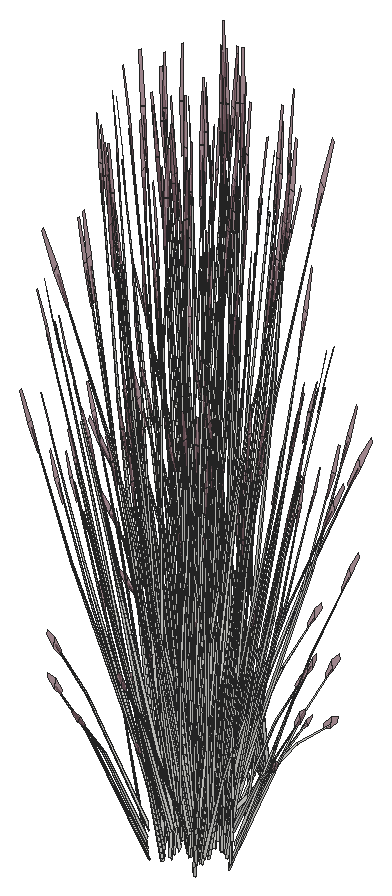
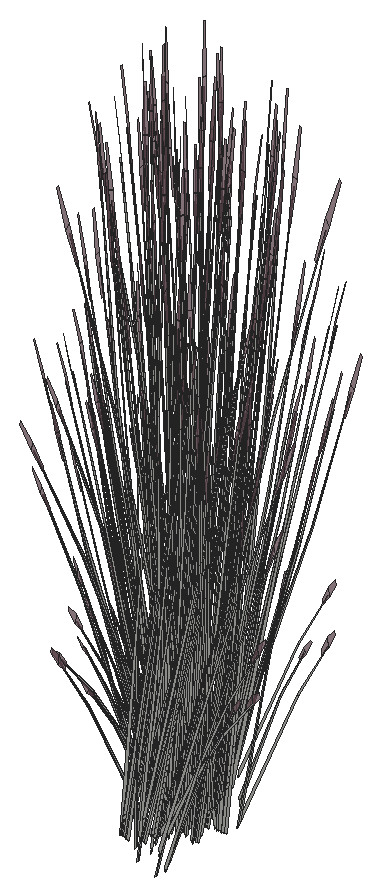
# SketchUp Ruby script. Lengths in inches.
U = 1.inch
M = Sketchup.active_model
def pt(a) = Geom::Point3d.new(a.map { |v| v * U })
def face(e, loops, mat)
  f = e.add_face(loops[0].map { |a| pt(a) })
  loops[1..].each { |l| e.add_face(l.map { |a| pt(a) }).erase! }
  f.material = f.back_material = mat if mat
  f
end
# faces: each face lists its corners as indices into pts; further lists are holes
def faces(e, pts, list, mat = nil) = list.each { |f| face(e, (f[0].is_a?(Array) ? f : [f]).map { |l| l.map { |i| pts[i] } }, mat) }
# xy, xz, yz: faces in a plane at the given z, y or x. An outline is a flat list of corners, or four numbers for a rectangle; further outlines are holes
def ring(l) = l.size == 4 ? [[l[0], l[1]], [l[2], l[1]], [l[2], l[3]], [l[0], l[3]]] : l.each_slice(2).to_a
def flat(e, list, mat, &to3) = list.each { |f| face(e, (f[0].is_a?(Array) ? f : [f]).map { |l| ring(l).map { |u, v| to3.(u, v) } }, mat) }
def xy(e, z, list, mat = nil) = flat(e, list, mat) { |x, y| [x, y, z] }
def xz(e, y, list, mat = nil) = flat(e, list, mat) { |x, z| [x, y, z] }
def yz(e, x, list, mat = nil) = flat(e, list, mat) { |y, z| [x, y, z] }
def lines(e, pts, list) = list.each { |a, b| e.add_line(pt(pts[a]), pt(pts[b])) }
# prism: a flat outline (further loops are holes) pulled along v
def prism(e, loops, v, mat = nil)
  f = face(e, loops, mat); d = Geom::Vector3d.new(v.map { |x| x * U })
  f.pushpull(f.normal.samedirection?(d) ? d.length : -d.length)
end
def box(e, o, s, mat = nil) = prism(e, [[o, [o[0] + s[0], o[1], o[2]], [o[0] + s[0], o[1] + s[1], o[2]], [o[0], o[1] + s[1], o[2]]]], [0, 0, s[2]], mat)
def at(x, y, z, deg = 0) = Geom::Transformation.translation(pt([x, y, z])) * Geom::Transformation.rotation(ORIGIN, Z_AXIS, deg.degrees)
def axes(o, x, y, z) = Geom::Transformation.new([*x, 0, *y, 0, *z, 0, *pt(o).to_a, 1])
def part(name) = M.definitions.add(name)
# library, detail: a bought-in or finely detailed component or shape, given as its bounding box
def library(name, o, s) = part(name).tap { |d| box(d.entities, o, s) }
def detail(e, o, s) = box(e.add_group.entities, o, s)
def put(e, d, t, mat = nil) = e.add_instance(d, t).tap { |i| i.material = mat if mat }
def group(e, t, mat = nil) = e.add_group.tap { |g| g.transformation = t; g.material = mat if mat }.entities
root = M.entities
M.materials.add("LightPink_Translucent").color = [144, 107, 117]
M.materials["LightPink_Translucent"].alpha = 0.75
c1 = part("blade")
p = [[2.15,0.21,22],[0,0.17,0],[0.09,0.45,0],[2.18,0.31,22],[2.29,0.31,22],[0.38,0.45,0],
  [2.48,0.24,33],[2.49,0.24,33],[2.48,0.22,33]]
faces(c1.entities,p,[[0,1,2,3],[4,5,2,3],[6,3,4,7],[8,0,3,6]])
c2 = part("seeds")
p = [[0.3,-0.1,1.38],[-0.01,-0.03,1.59],[-0.01,-0.03,0.03],[0.14,-0.07,-0.07],[0.29,-0.03,3],[0.15,0.01,3.11]]
faces(c2.entities,p,[[0,1,2,3],[1,0,4,5]],"LightPink_Translucent")
c3 = part("blade with seeds")
put(c3.entities,c1,at(0,0,0))
put(c3.entities,c2,axes([2.4,0.25,30.99],[1.5799,-0.05474,1.17369],[-0.12525,1.92788,0.29478],[-0.07173,-0.02425,1.56792]))
put(root,c3,axes([413.03,278.98,-8.39],[-0.09522,0.18683,1.59586],[-0.39947,-0.38663,0.12904],[0.18021,-0.24097,0.68222]))
put(root,c3,axes([414.33,278.06,-7.62],[-0.05194,0.04152,1.65179],[-0.50886,-0.14007,-0.15608],[-0.01842,-0.18118,0.29231]))
put(root,c3,axes([412.46,278.72,-7.64],[-0.50273,-0.13626,-0.47583],[0.17232,-0.46717,-0.36857],[-0.0461,-0.18809,0.91046]))
put(root,c3,axes([412.77,277.55,-9.42],[0.06561,0.31695,1.06958],[-0.36394,-0.17555,0.78586],[0.03916,-0.16229,0.23558]))
put(root,c3,axes([413.55,279.07,-7.64],[-0.3661,-0.36521,-0.47583],[0.38674,-0.31985,-0.36857],[0.0557,-0.18556,0.91046]))
put(root,c3,axes([411.5625,277.27,-7.62],[-0.00954,0.06515,1.65179],[-0.47055,0.23645,-0.15608],[-0.13847,-0.12087,0.29231]))
put(root,c3,axes([411.46,278.43,-7.26],[0.56969,-0.13971,0.50064],[0.09887,0.54803,0.4128],[-0.13398,-0.16152,1.03595]))
put(root,c3,axes([412.75,278.53,-7.59],[0.50393,0.1421,0.447],[-0.17232,0.46717,0.36857],[-0.03028,-0.18372,0.92496]))
put(root,c3,axes([412.89,278.7,-7.3125],[-0.50045,0.25306,-0.11324],[-0.24593,-0.44915,-0.62851],[-0.06603,-0.18927,0.95501]))
put(root,c3,axes([413.93,279.26,-7.3125],[-0.56206,-0.02693,-0.11324],[0.01536,-0.50991,-0.62851],[0.03904,-0.19638,0.95501]))
put(root,c3,axes([413.89,278.9375,-7.78],[0.34603,-0.28618,-0.32977],[0.32756,0.32677,0.42575],[0.04984,-0.16603,0.81462]))
put(root,c3,axes([410.9,277.93,-9.42],[0.26677,0.18918,1.06958],[-0.38851,0.11372,0.78586],[-0.08313,-0.14539,0.23558]))
put(root,c3,axes([412.88,278.49,-7.6],[0.37684,-0.18473,0.05988],[0.18445,0.33686,0.47138],[-0.03639,-0.14849,0.71878]))
put(root,c3,axes([411.54,278.93,-7.36],[-0.43608,-0.26272,-0.66157],[0.30991,-0.46038,0.07984],[-0.158,-0.15687,0.93586]))
put(root,c3,axes([411.39,278.58,-7.78],[-0.07899,-0.43781,-0.32977],[0.45153,-0.11561,0.42575],[-0.12128,-0.12546,0.81462]))
put(root,c3,axes([411.59,278.54,-7.6],[0.23243,-0.34529,0.05988],[0.331,0.20103,0.47138],[-0.10701,-0.1107,0.71878]))
put(root,c3,axes([410.69,278.5,-10.61],[-0.04954,0.0716,1.6421],[-0.50062,0.15438,-0.25086],[-0.12094,-0.14044,0.2797]))
put(root,c3,axes([411.52,280.47,-10.05],[-0.21003,-0.55738,-0.65031],[0.60499,-0.20074,-0.17068],[-0.02321,-0.18874,1.43544]))
put(root,c3,axes([414.32,278.76,-10.61],[-0.07655,-0.04282,1.6421],[-0.19662,-0.47839,-0.25086],[0.13264,-0.12982,0.2797]))
put(root,c3,axes([412.74,278.87,-7.3],[-0.15418,0.41799,0.32977],[-0.44981,-0.12192,-0.42575],[-0.04124,-0.16829,0.81462]))
put(root,c3,axes([411.34,278.94,-7.64],[-0.50465,0.12921,-0.47583],[-0.08828,-0.48932,-0.36857],[-0.13555,-0.14022,0.91046]))
put(root,c3,axes([413.89,279.05,-7.59],[0.36417,0.37086,0.447],[-0.38674,0.31985,0.36857],[0.06718,-0.174,0.92496]))
put(root,c3,axes([411.69,278.51,-6.94],[-0.34131,0.52108,-0.12682],[-0.49429,-0.3002,-0.70393],[-0.17182,-0.14722,1.06961]))
put(root,c3,axes([414.02,279.08,-7.6],[0.42027,0.02533,0.05988],[-0.01152,0.38243,0.47138],[0.04398,-0.14649,0.71878]))
put(root,c3,axes([413.71,279.34,-7.3],[-0.34603,0.28618,0.32977],[-0.32756,-0.32677,-0.42575],[0.04984,-0.16603,0.81462]))
put(root,c3,axes([414.32,280.11,-7.36],[0.26714,-0.42887,-0.66157],[0.46811,0.30479,0.07984],[0.1595,-0.15539,0.93586]))
put(root,c3,axes([411.43,278.86,-9.79],[-0.31974,-0.54466,0],[0.53494,-0.30375,-0.48057],[0.12184,-0.06918,1.52448]))
put(root,c3,axes([414.31,279.91,-7.64],[-0.13138,-0.49631,-0.47583],[0.49754,-0.08682,-0.36857],[0.14258,-0.13331,0.91046]))
put(root,c3,axes([412.14,278.21,-10.02],[-0.35341,0.31182,-0.03625],[-0.32382,-0.34152,-0.16435],[-0.0228,-0.09677,0.54209]))
put(root,c3,axes([414.54,280.27,-7.3125],[-0.47307,-0.29971,-0.11324],[0.27254,-0.43404,-0.62851],[0.13365,-0.15087,0.95501]))
put(root,c3,axes([412.59,281.9,-8.9],[0.44194,0.21918,1.40854],[-0.43295,0.47219,0.557],[-0.19393,-0.27986,1.18082]))
put(root,c3,axes([411.66,278.94,-7.3],[0.07899,0.43781,0.32977],[-0.45153,0.11561,-0.42575],[-0.12128,-0.12546,0.81462]))
put(root,c3,axes([410.28,280.39,-10.12],[0,-0.54355,-0.46235],[0.57217,0,0],[0,-0.1238,1.46668]))
put(root,c3,axes([411.87,278.78,-10.12],[0.47863,-0.27177,-0.46235],[0.28609,0.48733,0],[0.10901,-0.0619,1.46668]))
put(root,c3,axes([414.71,279.72,-9.59],[-0.1827,-0.0161,1.33163],[-0.18717,-0.43188,-0.28638],[0.22444,-0.12218,0.56934]))
put(root,c3,axes([410.3,279.23,-7.26],[0.42234,-0.40113,0.50064],[0.36424,0.42599,0.4128],[-0.19815,-0.07399,1.03595]))
put(root,c3,axes([415.71,280.14,-7.62],[-0.0668,-0.00413,1.65179],[-0.27738,-0.44233,-0.15608],[0.11139,-0.14544,0.29231]))
put(root,c3,axes([412.44,279.89,-10.08],[0.34446,-0.40855,-0.58063],[0.42791,0.37046,-0.15239],[0.13803,-0.10191,1.28164]))
put(root,c3,axes([414.92,278.92,-9.42],[-0.17034,0.27669,1.06958],[-0.14642,-0.37174,0.78586],[0.14069,-0.09315,0.23558]))
put(root,c3,axes([414.68,279.96,-7.78],[0.44516,-0.07768,-0.32977],[0.11755,0.44407,0.42575],[0.12757,-0.11927,0.81462]))
put(root,c3,axes([410.5,279.22,-7.6],[0.02575,-0.41332,0.05988],[0.38885,0.01133,0.47138],[-0.14895,-0.04325,0.71878]))
put(root,c3,axes([411.84,280.61,-9.94],[0.24813,-0.48978,-0.41661],[0.51557,0.23571,0.2005],[0,-0.1129,1.33761]))
put(root,c3,axes([412.0625,280.37,-9.52],[-0.05959,-0.62022,-0.27094],[0.62068,-0.0375,-0.46562],[0.1093,-0.08261,1.4872]))
put(root,c3,axes([410.52,280.4,-10.11],[0.35699,-0.33913,-0.28847],[0.35699,0.33913,0.28847],[0,-0.10923,1.29413]))
put(root,c3,axes([410.38,278.77,-10.02],[-0.14753,0.44383,-0.03625],[-0.45406,-0.13653,-0.16435],[-0.06894,-0.07259,0.54209]))
put(root,c3,axes([414.3125,280.23,-7.3],[-0.44516,0.07768,0.32977],[-0.11755,-0.44407,-0.42575],[0.12757,-0.11927,0.81462]))
put(root,c3,axes([411.77,281.02,-9.52],[-0.57594,-0.25935,-0.27094],[0.27732,-0.5474,-0.46562],[-0.0181,-0.1344,1.4872]))
put(root,c3,axes([410.13,280.8,-9.79],[-0.63949,0,0],[0,-0.60749,-0.48057],[0,-0.13836,1.52448]))
put(root,c3,axes([411.98,278.99,-10.11],[0.47712,0.13449,-0.28847],[-0.12013,0.47362,0.28847],[0.09619,-0.05462,1.29413]))
put(root,c3,axes([414.72,280.16,-7.6],[0.35109,0.22859,0.05988],[-0.2044,0.32553,0.47138],[0.11256,-0.10524,0.71878]))
put(root,c3,axes([414.62,280.06,-7.59],[0.12683,0.50025,0.447],[-0.49754,0.08682,0.36857],[0.14663,-0.11765,0.92496]))
put(root,c3,axes([415.96,280.67,-7.61],[0.07097,-0.08279,1.62908],[-0.09083,-0.50786,-0.25764],[0.17806,-0.09629,0.13065]))
put(root,c3,axes([410.63,280.64,-9.83],[-0.47569,0.45698,0.2864],[-0.47598,-0.45217,-0.33981],[-0.01661,-0.12977,1.53541]))
put(root,c3,axes([412.14,280.85,-9.73],[0.57623,0.26344,0.22409],[-0.27732,0.5474,0.46562],[0,-0.12618,1.49497]))
put(root,c3,axes([411.92,281.59,-9.73],[0.13555,-0.64407,-0.21817],[0.64269,0.11227,0.47743],[-0.1123,-0.08895,1.45677]))
put(root,c3,axes([410.76,279.53,-7.3],[0.29098,0.34031,0.32977],[-0.33226,0.32215,-0.42575],[-0.16881,-0.04902,0.81462]))
put(root,c3,axes([411.96,280.49,-9.47],[-0.55535,0.03355,0.41661],[-0.05022,-0.55698,-0.2005],[0.09942,-0.05645,1.33761]))
put(root,c3,axes([410.52,280.89,-9.69],[0,0.54355,0.46235],[-0.57217,0,0],[0,-0.1238,1.46668]))
put(root,c3,axes([414.5625,281.4375,-7.3125],[-0.25732,-0.49218,-0.11324],[0.45669,-0.24187,-0.62851],[0.19245,-0.06494,0.95501]))
put(root,c3,axes([414.54,281.01,-7.64],[0.13855,-0.49442,-0.47583],[0.47502,0.16947,-0.36857],[0.19125,-0.04534,0.91046]))
put(root,c3,axes([413.79,279,-9.79],[0.31974,-0.54466,0],[0.53494,0.30375,-0.48057],[0.12184,0.06918,1.52448]))
put(root,c3,axes([411.875,281.33,-9.94],[-0.30722,-0.45622,-0.41661],[0.46535,-0.32126,0.2005],[-0.09942,-0.05645,1.33761]))
put(root,c3,axes([411.9375,280.6875,-9.8],[0.22235,0.6078,0.42607],[-0.63531,0.21135,0.16719],[0.00776,-0.11168,1.47927]))
put(root,c3,axes([415.05,281.15,-10.15],[-0.32938,0.06523,1.31842],[-0.05243,-0.51922,0.07547],[0.2307,-0.07859,0.75023]))
put(root,c3,axes([415.65,280.69,-9.89],[-0.31706,-0.34757,-0.06041],[0.34725,-0.31847,-0.27392],[0.09839,-0.02242,0.90349]))
put(root,c3,axes([411.83,281.17,-9.47],[-0.24813,0.48978,0.41661],[-0.51557,-0.23571,-0.2005],[0,-0.1129,1.33761]))
put(root,c3,axes([412.74,280.74,-9.95],[0,-0.62892,0],[0.63949,0,0],[0,0,1.6711]))
put(root,c3,axes([413.51,279.29,-9.69],[-0.47863,-0.27177,0.46235],[0.28609,-0.48733,0],[0.10901,0.0619,1.46668]))
put(root,c3,axes([414.45,281.19,-7.36],[0.44939,-0.24006,-0.66157],[0.25044,0.49415,0.07984],[0.21713,-0.05613,0.93586]))
put(root,c3,axes([411.6,281.51,-10.08],[-0.53199,-0.08911,-0.58063],[0.11226,-0.54969,-0.15239],[-0.15876,-0.06661,1.28164]))
put(root,c3,axes([412.43,280.34,-9.8],[-0.42403,0.49328,0.42607],[-0.50377,-0.43543,0.16719],[0.10223,-0.04923,1.47927]))
put(root,c3,axes([412.9,281.23,-9.86],[-0.47569,-0.46784,-0.05709],[0.47598,-0.46812,0],[-0.01661,-0.01634,1.63492]))
put(root,c3,axes([411.7,279.53,-9.7],[-0.14774,0.54019,0.16428],[-0.54062,-0.15287,0.32672],[0.09339,-0.00263,1.49371]))
put(root,c3,axes([414.38,281.29,-7.3],[-0.42502,-0.15163,0.32977],[0.12396,-0.44238,-0.42575],[0.17112,-0.04056,0.81462]))
put(root,c3,axes([411.47,279.97,-10.52],[-0.50338,0.21762,1.20058],[-0.16022,-0.62439,0.4665],[0.30911,0.01039,1.36553]))
put(root,c3,axes([412.83,280.13,-9.5625],[0.09866,-0.48509,0.13483],[0.48202,0.0842,-0.38503],[0.08772,0.04981,1.18024]))
put(root,c3,axes([411.99,281.28,-9.8],[0.64638,0.11452,0.42607],[-0.13155,0.64678,0.16719],[-0.09446,-0.06245,1.47927]))
put(root,c3,axes([415.41,280.8125,-10.61],[-0.02673,-0.08252,1.6421],[0.18538,-0.48271,-0.25086],[0.187,-0.00694,0.2797]))
put(root,c3,axes([412.62,280.26,-9.47],[-0.30722,-0.45622,0.41661],[0.46535,-0.32126,-0.2005],[0.09942,0.05645,1.33761]))
put(root,c3,axes([411.03,282.34,-10.11],[-0.12013,-0.47362,-0.28847],[0.47712,-0.13449,0.28847],[-0.09619,-0.05462,1.29413]))
put(root,c3,axes([411.65,282.32,-9.7],[0.54955,-0.14427,0.16428],[0.1357,0.53689,0.32672],[-0.04901,-0.07823,1.49371]))
put(root,c3,axes([412.78,280.29,-9.52],[0.51635,-0.36087,-0.27094],[0.34336,0.5099,-0.46562],[0.1274,0.05178,1.4872]))
put(root,c3,axes([414.83,281.24,-7.78],[0.42502,0.15163,-0.32977],[-0.12396,0.44238,0.42575],[0.17112,-0.04056,0.81462]))
put(root,c3,axes([410.9,282.55,-10.12],[-0.47863,-0.27177,-0.46235],[0.28609,-0.48733,0],[-0.10901,-0.0619,1.46668]))
put(root,c3,axes([414.08,279.33,-10.12],[0.47863,0.27177,-0.46235],[-0.28609,0.48733,0],[0.10901,0.0619,1.46668]))
put(root,c3,axes([413.17,280.88,-9.95],[0.57217,0,0],[0,0.56272,0],[0,0,1.66132]))
put(root,c3,axes([412.2,281.59,-9.52],[-0.51635,0.36087,-0.27094],[-0.34336,-0.5099,-0.46562],[-0.1274,-0.05178,1.4872]))
put(root,c3,axes([413.33,279.56,-9.7],[-0.54955,0.14427,0.16428],[-0.1357,-0.53689,0.32672],[0.04901,0.07823,1.49371]))
put(root,c3,axes([413.67,280.69,-8.39],[-0.21212,0.01231,1.59586],[0.14072,-0.53355,0.12904],[0.3023,0.033,0.68222]))
put(root,c3,axes([413.95,279.53,-10.11],[0.12013,0.47362,-0.28847],[-0.47712,0.13449,0.28847],[0.09619,0.05462,1.29413]))
put(root,c3,axes([414.77,281.43,-7.6],[0.18783,0.37061,0.05988],[-0.34252,0.1814,0.47138],[0.15099,-0.03579,0.71878]))
put(root,c3,axes([412.99,280.59,-9.78],[-0.64638,-0.11452,0.45814],[0.13155,-0.64678,0.17978],[0.09446,0.06245,1.59061]))
put(root,c3,axes([414.73,281.29,-7.59],[-0.14449,0.4956,0.447],[-0.47502,-0.16947,0.36857],[0.1868,-0.02978,0.92496]))
put(root,c3,axes([412.47,282.19,-9.95],[-0.16686,-0.46861,0],[0.47648,-0.16411,0],[0,0,1.4375]))
put(root,c3,axes([412.15,281.75,-9.5625],[-0.09866,0.48509,0.13483],[-0.48202,-0.0842,-0.38503],[-0.08772,-0.04981,1.18024]))
put(root,c3,axes([410.28,280.49,-7.3],[0.42502,0.15163,0.32977],[-0.12396,0.44238,-0.42575],[-0.17112,0.04056,0.81462]))
put(root,c3,axes([413.1,282.125,-9.97],[0.53691,-0.18442,-0.17877],[0.18866,0.53125,0.00007],[0.05927,-0.02038,1.61933]))
put(root,c3,axes([413.28,282.35,-9.7],[0.14774,-0.54019,0.16428],[0.54062,0.15287,0.32672],[-0.09339,0.00263,1.49371]))
put(root,c3,axes([413.16,281.12,-9.9375],[0.35699,0.35109,0],[-0.35699,0.35109,0],[0,0,1.57621]))
put(root,c3,axes([414.125,280.97,-9.7],[-0.40181,-0.39593,0.16428],[0.40492,-0.38402,0.32672],[-0.04438,0.08086,1.49371]))
put(root,c3,axes([413.38,280.37,-10.08],[0.53199,0.08911,-0.58063],[-0.11226,0.54969,-0.15239],[0.15876,0.06661,1.28164]))
put(root,c3,axes([415.73,281.33,-9.42],[-0.31598,0.08973,1.06958],[0.14873,-0.37085,0.78586],[0.16763,0.02538,0.23558]))
put(root,c3,axes([412.35,282.4,-9.95],[-0.51557,-0.24403,0],[0.24813,-0.50705,0],[0,0,1.51513]))
put(root,c3,axes([412.78,281.75,-9.7],[-0.49938,-0.43748,-0.23459],[0.42021,-0.49126,0.51337],[-0.13447,0.05118,1.56642]))
put(root,c3,axes([411.47,282.59,-9.69],[0.47863,0.27177,0.46235],[-0.28609,0.48733,0],[-0.10901,-0.0619,1.46668]))
put(root,c3,axes([413.15,280.71,-9.47],[0.24813,-0.48978,0.41661],[0.51557,0.23571,-0.2005],[0,0.1129,1.33761]))
put(root,c3,axes([415.59,282.9,-7.62],[-0.04624,-0.04758,1.65179],[0.10116,-0.51007,-0.15608],[0.18215,-0.03259,0.29231]))
put(root,c3,axes([413.06,280.99,-9.87],[0,0.62861,-0.05249],[-0.63949,0,0],[0,0.01975,1.67027]))
put(root,c3,axes([413.11,280.54,-9.94],[0.30722,0.45622,-0.41661],[-0.46535,0.32126,0.2005],[0.09942,0.05645,1.33761]))
put(root,c3,axes([415.18,282.47,-8.34],[-0.09788,-0.45691,-0.03251],[0.46264,-0.10504,-0.14742],[0.09661,0.02897,0.48626]))
put(root,c3,axes([411.19,282.875,-9.79],[-0.31974,0.54466,0],[-0.53494,-0.30375,-0.48057],[-0.12184,-0.06918,1.52448]))
put(root,c3,axes([413.98,282.46,-7.3125],[0.02738,-0.55277,-0.11324],[0.51847,0.01511,-0.62851],[0.19968,0.0384,0.95501]))
put(root,c3,axes([414.46,280.98,-9.69],[0,-0.54355,0.46235],[0.57217,0,0],[0,0.1238,1.46668]))
put(root,c3,axes([413.02,281.39,-9.47],[0.55535,-0.03355,0.41661],[0.05022,0.55698,-0.2005],[-0.09942,0.05645,1.33761]))
put(root,c3,axes([413.37,280.82,-9.5625],[0.47648,-0.15851,0.13483],[0.16686,0.45265,-0.38503],[0,0.09962,1.18024]))
put(root,c3,axes([413.9,282.24,-7.3],[-0.29098,-0.34031,0.32977],[0.33226,-0.32215,-0.42575],[0.16881,0.04902,0.81462]))
put(root,c3,axes([412.53,281.66,-9.94],[-0.55535,0.03355,-0.41661],[-0.05022,-0.55698,0.2005],[-0.09942,0.05645,1.33761]))
put(root,c3,axes([415.14,281.92,-9.59],[-0.12317,-0.13368,1.33163],[0.16025,-0.44223,-0.28638],[0.24919,0.05991,0.56934]))
put(root,c3,axes([412.9375,282.41,-9.95],[0.51557,0.24403,0],[-0.24813,0.50705,0],[0,0,1.62917]))
put(root,c3,axes([414.43,282.13,-7.61],[0.10971,-0.00919,1.62908],[0.30091,-0.42228,-0.25764],[0.19514,0.05574,0.13065]))
put(root,c3,axes([413.14,282.95,-9.96],[-0.31576,-0.54657,-0.04789],[0.53494,-0.30375,0.48057],[-0.13182,0.05204,1.52373]))
put(root,c3,axes([413.03,281.63,-9.5625],[0.37783,0.32657,0.13483],[-0.31516,0.36844,-0.38503],[-0.08772,0.04981,1.18024]))
put(root,c3,axes([410.05,281.71,-7.59],[-0.12683,-0.50025,0.447],[0.49754,-0.08682,0.36857],[-0.14663,0.11765,0.92496]))
put(root,c3,axes([409.95,281.62,-7.6],[-0.35109,-0.22859,0.05988],[0.2044,-0.32553,0.47138],[-0.11256,0.10524,0.71878]))
put(root,c3,axes([409.8,287.9375,-8.39],[0.1169,0.17452,1.59586],[-0.54019,0.14692,0.12904],[-0.12209,-0.27397,0.68222]))
put(root,c3,axes([414.01,282.19,-7.36],[0.51122,0.01309,-0.66157],[-0.03434,0.5511,0.07984],[0.21658,0.05816,0.93586]))
put(root,c3,axes([410.69,286.78,-7.61],[-0.07822,-0.07621,1.62908],[-0.52201,0.04832,-0.25764],[-0.08331,-0.18228,0.13065]))
put(root,c3,axes([413.43,282.64,-9.69],[0.47863,-0.27177,0.46235],[0.28609,0.48733,0],[-0.10901,0.0619,1.46668]))
put(root,c3,axes([411.91,287.68,-9.59],[-0.14537,0.11002,1.33163],[-0.43536,-0.19256,-0.28638],[0.0807,-0.23948,0.56934]))
put(root,c3,axes([411.24,288.07,-7.36],[-0.24409,-0.44196,-0.66157],[0.50245,-0.2463,0.07984],[-0.05708,-0.21354,0.93586]))
put(root,c3,axes([412.75,282.21,-9.87],[0.22235,0.62444,-0.05599],[-0.63531,0.21881,0],[0.00776,0.02181,1.60327]))
put(root,c3,axes([413,282.88,-10.11],[-0.47712,-0.13449,-0.28847],[0.12013,-0.47362,0.28847],[-0.09619,0.05462,1.29413]))
put(root,c3,axes([409.65,287.48,-9.59],[-0.03097,0.17781,1.33163],[-0.45273,0.14885,-0.28638],[-0.10583,-0.22982,0.56934]))
put(root,c3,axes([410.35,281.55,-7.3],[0.44516,-0.07768,0.32977],[0.11755,0.44407,-0.42575],[-0.12757,0.11927,0.81462]))
put(root,c3,axes([414.84,281.08,-9.79],[0.63949,0,0],[0,0.60749,-0.48057],[0,0.13836,1.52448]))
put(root,c3,axes([410.82,287.09,-10.61],[-0.08578,0.01958,1.6421],[-0.47437,-0.22044,-0.25086],[0.00796,-0.18387,0.2797]))
put(root,c3,axes([414.59,281.39,-9.95],[-0.63917,-0.00435,-0.04634],[0,-0.60749,0.46507],[-0.02009,0.13829,1.47457]))
put(root,c3,axes([413.21,280.86,-9.52],[0.57594,0.25935,-0.27094],[-0.27732,0.5474,-0.46562],[0.0181,0.1344,1.4872]))
put(root,c3,axes([414.32,282.42,-7.78],[0.29098,0.34031,-0.32977],[-0.33226,0.32215,0.42575],[0.16881,0.04902,0.81462]))
put(root,c3,axes([414.46,281.48,-10.11],[-0.35699,0.33913,-0.28847],[-0.35699,-0.33913,0.28847],[0,0.10923,1.29413]))
put(root,c3,axes([412.92,281.51,-9.52],[0.05959,0.62022,-0.27094],[-0.62068,0.0375,-0.46562],[-0.1093,0.08261,1.4872]))
put(root,c3,axes([412.26,288.5,-7.36],[0.01331,-0.50278,-0.66157],[0.56035,0.03377,0.07984],[0.05914,-0.213,0.93586]))
put(root,c3,axes([414.17,282.55,-7.6],[-0.02575,0.41332,0.05988],[-0.38885,-0.01133,0.47138],[0.14895,0.04325,0.71878]))
put(root,c3,axes([413.14,281.27,-9.94],[-0.24813,0.48978,-0.41661],[-0.51557,-0.23571,0.2005],[0,0.1129,1.33761]))
put(root,c3,axes([414.2,282.42,-7.59],[-0.37709,0.35815,0.447],[-0.32522,-0.38035,0.36857],[0.17692,0.06607,0.92496]))
put(root,c3,axes([413.04,287.71,-7.61],[-0.00494,-0.10818,1.62908],[-0.41695,-0.31265,-0.25764],[0.06446,-0.18952,0.13065]))
put(root,c3,axes([411.29,287.69,-7.78],[0.15418,-0.41799,-0.32977],[0.44981,0.12192,0.42575],[-0.04124,-0.16829,0.81462]))
put(root,c3,axes([411.63,288.24,-8.39],[-0.09522,0.18683,1.59586],[-0.39947,-0.38663,0.12904],[0.18021,-0.24097,0.68222]))
put(root,c3,axes([412.93,287.33,-7.62],[-0.05194,0.04152,1.65179],[-0.50886,-0.14007,-0.15608],[-0.01842,-0.18118,0.29231]))
put(root,c3,axes([411.06,287.98,-7.64],[-0.50273,-0.13626,-0.47583],[0.17232,-0.46717,-0.36857],[-0.0461,-0.18809,0.91046]))
put(root,c3,axes([411.37,286.81,-9.42],[0.06561,0.31695,1.06958],[-0.36394,-0.17555,0.78586],[0.03916,-0.16229,0.23558]))
put(root,c3,axes([409.34,282.81,-6.74],[0.45129,0.14509,-0.06041],[-0.13882,0.44656,-0.27392],[-0.07381,0.0678,0.90349]))
put(root,c3,axes([412.54,281.98,-10.08],[-0.34446,0.40855,-0.58063],[-0.42791,-0.37046,-0.15239],[-0.13803,0.10191,1.28164]))
put(root,c3,axes([412.15,288.33,-7.64],[-0.3661,-0.36521,-0.47583],[0.38674,-0.31985,-0.36857],[0.0557,-0.18556,0.91046]))
put(root,c3,axes([413,282.83,-7.3],[-0.07899,-0.43781,0.32977],[0.45153,-0.11561,-0.42575],[0.12128,0.12546,0.81462]))
put(root,c3,axes([410.16,286.53,-7.62],[-0.00954,0.06515,1.65179],[-0.47055,0.23645,-0.15608],[-0.13847,-0.12087,0.29231]))
put(root,c3,axes([413.16,282.67,-9.83],[0.64025,0.17667,0.2864],[-0.16018,0.63149,-0.33981],[-0.10597,0.07904,1.53541]))
put(root,c3,axes([413.11,283.1,-10.12],[-0.47863,0.27177,-0.46235],[-0.28609,-0.48733,0],[-0.10901,0.0619,1.46668]))
put(root,c3,axes([414.7,281.49,-10.12],[0,0.54355,-0.46235],[-0.57217,0,0],[0,0.1238,1.46668]))
put(root,c3,axes([413.27,281.55,-8.39],[-0.18996,-0.09365,1.59586],[0.39312,-0.39287,0.12904],[0.24502,0.17723,0.68222]))
put(root,c3,axes([413.31,280.32,-7.83],[-0.44191,-0.28242,1.28769],[0.46662,-0.43971,0.5556],[0.14258,0.26499,1.24467]))
put(root,c3,axes([410.06,287.6875,-7.26],[0.56969,-0.13971,0.50064],[0.09887,0.54803,0.4128],[-0.13398,-0.16152,1.03595]))
put(root,c3,axes([410.12,281.51,-7.3125],[0.47307,0.29971,-0.11324],[-0.27254,0.43404,-0.62851],[-0.13365,0.15087,0.95501]))
put(root,c3,axes([411.34,287.79,-7.59],[0.50393,0.1421,0.447],[-0.17232,0.46717,0.36857],[-0.03028,-0.18372,0.92496]))
put(root,c3,axes([413.98,282.62,-9.42],[-0.28795,-0.15629,1.06958],[0.37181,-0.1588,0.78586],[0.10029,0.13452,0.23558]))
put(root,c3,axes([411.49,287.96,-7.3125],[-0.50045,0.25306,-0.11324],[-0.24593,-0.44915,-0.62851],[-0.06603,-0.18927,0.95501]))
put(root,c3,axes([412.53,288.52,-7.3125],[-0.56206,-0.02693,-0.11324],[0.01536,-0.50991,-0.62851],[0.03904,-0.19638,0.95501]))
put(root,c3,axes([412.96,283.0625,-7.3125],[0.30474,-0.46525,-0.11324],[0.44133,0.26804,-0.62851],[0.15341,0.13145,0.95501]))
put(root,c3,axes([412.49,288.2,-7.78],[0.34603,-0.28618,-0.32977],[0.32756,0.32677,0.42575],[0.04984,-0.16603,0.81462]))
put(root,c3,axes([409.5,287.19,-9.42],[0.26677,0.18918,1.06958],[-0.38851,0.11372,0.78586],[-0.08313,-0.14539,0.23558]))
put(root,c3,axes([411.48,287.75,-7.6],[0.37684,-0.18473,0.05988],[0.18445,0.33686,0.47138],[-0.03639,-0.14849,0.71878]))
put(root,c3,axes([409.99,287.85,-7.78],[-0.07899,-0.43781,-0.32977],[0.45153,-0.11561,0.42575],[-0.12128,-0.12546,0.81462]))
put(root,c3,axes([410.36,281.86,-7.64],[0.13138,0.49631,-0.47583],[-0.49754,0.08682,-0.36857],[-0.14258,0.13331,0.91046]))
put(root,c3,axes([410.95,282.43,-7.3],[0.34603,-0.28618,0.32977],[0.32756,0.32677,-0.42575],[-0.04984,0.16603,0.81462]))
put(root,c3,axes([413.55,283.01,-9.79],[0.31974,0.54466,0],[-0.53494,0.30375,-0.48057],[-0.12184,0.06918,1.52448]))
put(root,c3,axes([412.56,283.45,-7.62],[0.00151,-0.06581,1.65179],[0.43826,-0.29033,-0.15608],[0.15223,0.10363,0.29231]))
put(root,c3,axes([414.06,283.2,-10.61],[0.03726,-0.07847,1.6421],[0.46909,-0.23111,-0.25086],[0.14221,0.11962,0.2797]))
put(root,c3,axes([413.27,280.86,-9.35],[-0.01397,-0.51177,1.31553],[0.63227,0.13266,0.557],[-0.14954,0.28003,1.24175]))
put(root,c3,axes([413.4375,281.41,-10.05],[0.18752,0.49766,-0.6445],[-0.54017,0.17923,-0.16915],[0.02073,0.16852,1.42262]))
